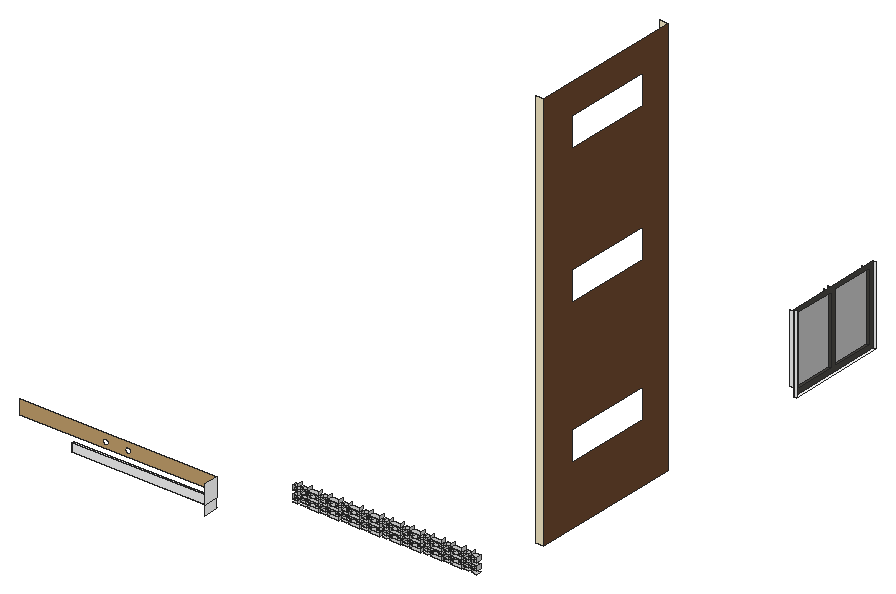
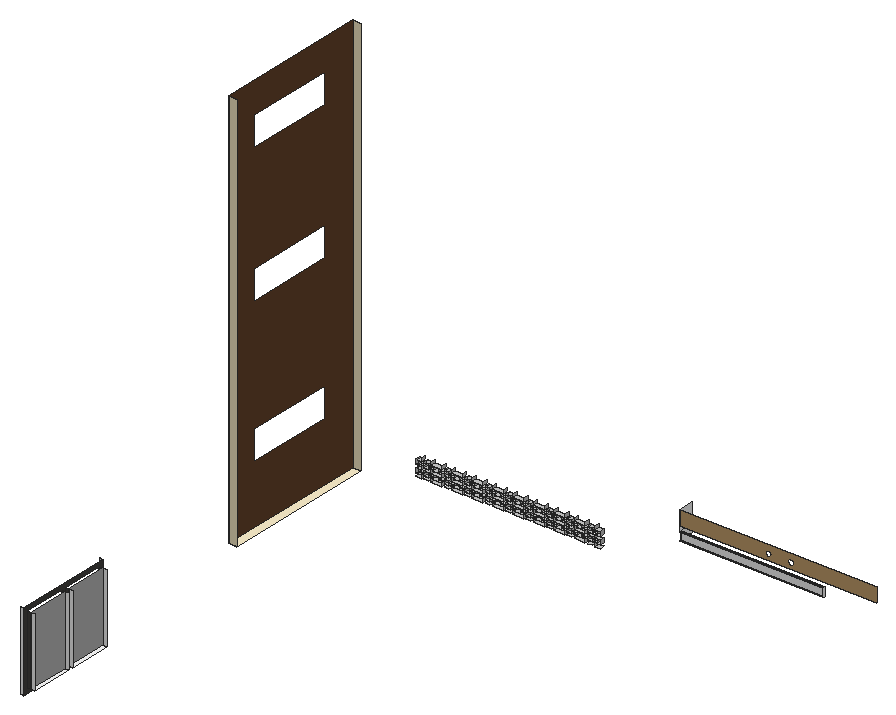
# SketchUp Ruby script. Lengths in inches.
U = 1.inch
M = Sketchup.active_model
def pt(a) = Geom::Point3d.new(a.map { |v| v * U })
def face(e, loops, mat)
  f = e.add_face(loops[0].map { |a| pt(a) })
  loops[1..].each { |l| e.add_face(l.map { |a| pt(a) }).erase! }
  f.material = f.back_material = mat if mat
  f
end
# faces: each face lists its corners as indices into pts; further lists are holes
def faces(e, pts, list, mat = nil) = list.each { |f| face(e, (f[0].is_a?(Array) ? f : [f]).map { |l| l.map { |i| pts[i] } }, mat) }
# xy, xz, yz: faces in a plane at the given z, y or x. An outline is a flat list of corners, or four numbers for a rectangle; further outlines are holes
def ring(l) = l.size == 4 ? [[l[0], l[1]], [l[2], l[1]], [l[2], l[3]], [l[0], l[3]]] : l.each_slice(2).to_a
def flat(e, list, mat, &to3) = list.each { |f| face(e, (f[0].is_a?(Array) ? f : [f]).map { |l| ring(l).map { |u, v| to3.(u, v) } }, mat) }
def xy(e, z, list, mat = nil) = flat(e, list, mat) { |x, y| [x, y, z] }
def xz(e, y, list, mat = nil) = flat(e, list, mat) { |x, z| [x, y, z] }
def yz(e, x, list, mat = nil) = flat(e, list, mat) { |y, z| [x, y, z] }
def lines(e, pts, list) = list.each { |a, b| e.add_line(pt(pts[a]), pt(pts[b])) }
# prism: a flat outline (further loops are holes) pulled along v
def prism(e, loops, v, mat = nil)
  f = face(e, loops, mat); d = Geom::Vector3d.new(v.map { |x| x * U })
  f.pushpull(f.normal.samedirection?(d) ? d.length : -d.length)
end
def box(e, o, s, mat = nil) = prism(e, [[o, [o[0] + s[0], o[1], o[2]], [o[0] + s[0], o[1] + s[1], o[2]], [o[0], o[1] + s[1], o[2]]]], [0, 0, s[2]], mat)
def at(x, y, z, deg = 0) = Geom::Transformation.translation(pt([x, y, z])) * Geom::Transformation.rotation(ORIGIN, Z_AXIS, deg.degrees)
def axes(o, x, y, z) = Geom::Transformation.new([*x, 0, *y, 0, *z, 0, *pt(o).to_a, 1])
def part(name) = M.definitions.add(name)
# library, detail: a bought-in or finely detailed component or shape, given as its bounding box
def library(name, o, s) = part(name).tap { |d| box(d.entities, o, s) }
def detail(e, o, s) = box(e.add_group.entities, o, s)
def put(e, d, t, mat = nil) = e.add_instance(d, t).tap { |i| i.material = mat if mat }
def group(e, t, mat = nil) = e.add_group.tap { |g| g.transformation = t; g.material = mat if mat }.entities
root = M.entities
M.materials.add("D01_Frost_White").color = [255, 242, 206]
M.materials.add("Glass_Mirror_01").color = [185, 185, 185]
M.materials.add("M00_Soft_Cloud").color = [255, 255, 255]
M.materials.add("Metal_Perforated_03_1K").color = [205, 205, 205]
M.materials.add("Plywood_08_1K").color = [202, 166, 113]
M.materials.add("Wood_Planks_01_1K").color = [69, 67, 63]
M.materials.add("Wood_Veneer_15_1K1").color = [103, 69, 45]
xy(root,36.13,[[230.81,76.77,353.54,78.27]],"M00_Soft_Cloud")
xy(root,36.14,[[388.18,115.4375,392.79,119.17],[401.01,115.4375,410.24,119.17],[418.47,115.4375,427.69,119.17],[435.92,115.4375,445.15,119.17],[453.37,115.4375,462.6,119.17],
  [470.82,115.4375,480.05,119.17],[488.27,115.4375,497.5,119.17],[505.72,115.4375,514.95,119.17],[523.18,115.4375,532.4,119.17],[540.63,115.4375,545.24,119.17]],"Metal_Perforated_03_1K")
xy(root,36.25,[[394.84,115.4375,398.97,119.17],[412.29,115.4375,416.42,119.17],[429.74,115.4375,433.87,119.17],[447.19,115.4375,451.32,119.17],[464.65,115.4375,468.77,119.17],
  [482.1,115.4375,486.22,119.17],[499.55,115.4375,503.68,119.17],[517,115.4375,521.13,119.17],[534.45,115.4375,538.58,119.17]],"Metal_Perforated_03_1K")
xy(root,38.1,[[561.28,433.07,564,517.74]],"M00_Soft_Cloud")
xy(root,38.71,[[394.84,115.4375,398.97,119.17],[412.29,115.4375,416.42,119.17],[429.74,115.4375,433.87,119.17],[447.19,115.4375,451.32,119.17],[464.65,115.4375,468.77,119.17],
  [482.1,115.4375,486.22,119.17],[499.55,115.4375,503.68,119.17],[517,115.4375,521.13,119.17],[534.45,115.4375,538.58,119.17]],"Metal_Perforated_03_1K")
xy(root,38.8125,[[388.18,115.4375,392.79,119.17],[401.01,115.4375,410.24,119.17],[418.47,115.4375,427.69,119.17],[435.92,115.4375,445.15,119.17],[453.37,115.4375,462.6,119.17],
  [470.82,115.4375,480.05,119.17],[488.27,115.4375,497.5,119.17],[505.72,115.4375,514.95,119.17],[523.18,115.4375,532.4,119.17],[540.63,115.4375,545.24,119.17]],"Metal_Perforated_03_1K")
xy(root,40.05,[[390.22,115.4375,394.84,119.17],[398.97,115.4375,403.58,119.17],[407.68,115.4375,412.29,119.17],[416.42,115.4375,421.03,119.17],[425.13,115.4375,429.74,119.17],
  [433.87,115.4375,438.48,119.17],[442.58,115.4375,447.19,119.17],[451.32,115.4375,455.93,119.17],[460.03,115.4375,464.65,119.17],[468.77,115.4375,473.39,119.17],
  [477.48,115.4375,482.1,119.17],[486.22,115.4375,490.84,119.17],[494.94,115.4375,499.55,119.17],[503.68,115.4375,508.29,119.17],[512.39,115.4375,517,119.17],
  [521.13,115.4375,525.74,119.17],[529.84,115.4375,534.45,119.17],[538.58,115.4375,543.19,119.17]],"Metal_Perforated_03_1K")
xy(root,41.4,[[390.22,115.4375,394.84,119.17],[398.97,115.4375,403.58,119.17],[407.68,115.4375,412.29,119.17],[416.42,115.4375,421.03,119.17],[425.13,115.4375,429.74,119.17],
  [433.87,115.4375,438.48,119.17],[442.58,115.4375,447.19,119.17],[451.32,115.4375,455.93,119.17],[460.03,115.4375,464.65,119.17],[468.77,115.4375,473.39,119.17],
  [477.48,115.4375,482.1,119.17],[486.22,115.4375,490.84,119.17],[494.94,115.4375,499.55,119.17],[503.68,115.4375,508.29,119.17],[512.39,115.4375,517,119.17],
  [521.13,115.4375,525.74,119.17],[529.84,115.4375,534.45,119.17],[538.58,115.4375,543.19,119.17]],"Metal_Perforated_03_1K")
xy(root,42.1,[[555,437.07,558.14,473.4],[555,477.4,558.14,513.74]],"M00_Soft_Cloud")
xy(root,42.1,[[558.14,437.07,561.28,473.4],[558.14,477.4,561.28,513.74]],"Wood_Planks_01_1K")
xy(root,42.64,[[388.18,115.4375,392.79,119.17],[401.01,115.4375,410.24,119.17],[418.47,115.4375,427.69,119.17],[435.92,115.4375,445.15,119.17],[453.37,115.4375,462.6,119.17],
  [470.82,115.4375,480.05,119.17],[488.27,115.4375,497.5,119.17],[505.72,115.4375,514.95,119.17],[523.18,115.4375,532.4,119.17],[540.63,115.4375,545.24,119.17]],"Metal_Perforated_03_1K")
xy(root,42.74,[[394.84,115.4375,398.97,119.17],[412.29,115.4375,416.42,119.17],[429.74,115.4375,433.87,119.17],[447.19,115.4375,451.32,119.17],[464.65,115.4375,468.77,119.17],
  [482.1,115.4375,486.22,119.17],[499.55,115.4375,503.68,119.17],[517,115.4375,521.13,119.17],[534.45,115.4375,538.58,119.17]],"Metal_Perforated_03_1K")
xy(root,43.27,[[230.81,76.77,353.54,78.27]],"M00_Soft_Cloud")
xy(root,45.2,[[394.84,115.4375,398.97,119.17],[412.29,115.4375,416.42,119.17],[429.74,115.4375,433.87,119.17],[447.19,115.4375,451.32,119.17],[464.65,115.4375,468.77,119.17],
  [482.1,115.4375,486.22,119.17],[499.55,115.4375,503.68,119.17],[517,115.4375,521.13,119.17],[534.45,115.4375,538.58,119.17]],"Metal_Perforated_03_1K")
xy(root,45.31,[[388.18,115.4375,392.79,119.17],[401.01,115.4375,410.24,119.17],[418.47,115.4375,427.69,119.17],[435.92,115.4375,445.15,119.17],[453.37,115.4375,462.6,119.17],
  [470.82,115.4375,480.05,119.17],[488.27,115.4375,497.5,119.17],[505.72,115.4375,514.95,119.17],[523.18,115.4375,532.4,119.17],[540.63,115.4375,545.24,119.17]],"Metal_Perforated_03_1K")
xy(root,46.54,[[390.22,115.4375,394.84,119.17],[398.97,115.4375,403.58,119.17],[407.68,115.4375,412.29,119.17],[416.42,115.4375,421.03,119.17],[425.13,115.4375,429.74,119.17],
  [433.87,115.4375,438.48,119.17],[442.58,115.4375,447.19,119.17],[451.32,115.4375,455.93,119.17],[460.03,115.4375,464.65,119.17],[468.77,115.4375,473.39,119.17],
  [477.48,115.4375,482.1,119.17],[486.22,115.4375,490.84,119.17],[494.94,115.4375,499.55,119.17],[503.68,115.4375,508.29,119.17],[512.39,115.4375,517,119.17],
  [521.13,115.4375,525.74,119.17],[529.84,115.4375,534.45,119.17],[538.58,115.4375,543.19,119.17]],"Metal_Perforated_03_1K")
xy(root,47.9,[[390.22,115.4375,394.84,119.17],[398.97,115.4375,403.58,119.17],[407.68,115.4375,412.29,119.17],[416.42,115.4375,421.03,119.17],[425.13,115.4375,429.74,119.17],
  [433.87,115.4375,438.48,119.17],[442.58,115.4375,447.19,119.17],[451.32,115.4375,455.93,119.17],[460.03,115.4375,464.65,119.17],[468.77,115.4375,473.39,119.17],
  [477.48,115.4375,482.1,119.17],[486.22,115.4375,490.84,119.17],[494.94,115.4375,499.55,119.17],[503.68,115.4375,508.29,119.17],[512.39,115.4375,517,119.17],
  [521.13,115.4375,525.74,119.17],[529.84,115.4375,534.45,119.17],[538.58,115.4375,543.19,119.17]],"Metal_Perforated_03_1K")
xy(root,49.13,[[388.18,115.4375,392.79,119.17],[401.01,115.4375,410.24,119.17],[418.47,115.4375,427.69,119.17],[435.92,115.4375,445.15,119.17],[453.37,115.4375,462.6,119.17],
  [470.82,115.4375,480.05,119.17],[488.27,115.4375,497.5,119.17],[505.72,115.4375,514.95,119.17],[523.18,115.4375,532.4,119.17],[540.63,115.4375,545.24,119.17]],"Metal_Perforated_03_1K")
xy(root,49.23,[[394.84,115.4375,398.97,119.17],[412.29,115.4375,416.42,119.17],[429.74,115.4375,433.87,119.17],[447.19,115.4375,451.32,119.17],[464.65,115.4375,468.77,119.17],
  [482.1,115.4375,486.22,119.17],[499.55,115.4375,503.68,119.17],[517,115.4375,521.13,119.17],[534.45,115.4375,538.58,119.17]],"Metal_Perforated_03_1K")
xy(root,49.46,[[564,154.61,571,286.54]],"D01_Frost_White")
xz(root,76.77,[[230.81,36.13,353.54,43.27]],"M00_Soft_Cloud")
xz(root,78.27,[[[185.54,48,353.54,60],[258.34,50.6,257.72,50.68,257.14,50.92,256.65,51.3,256.27,51.8,256.03,52.38,255.94,53,256.03,53.62,256.27,54.2,256.65,54.7,257.14,55.08,257.72,55.32,258.34,55.4,258.97,55.32,259.54,55.08,260.04,54.7,260.42,54.2,260.66,53.62,260.74,53,260.66,52.38,260.42,51.8,260.04,51.3,259.54,50.92,258.97,50.68],[277.47,50.6,276.85,50.68,276.27,50.92,275.78,51.3,275.39,51.8,275.15,52.38,275.07,53,275.15,53.62,275.39,54.2,275.78,54.7,276.27,55.08,276.85,55.32,277.47,55.4,278.09,55.32,278.67,55.08,279.17,54.7,279.55,54.2,279.79,53.62,279.87,53,279.79,52.38,279.55,51.8,279.17,51.3,278.67,50.92,278.09,50.68]]],"Plywood_08_1K")
xz(root,154.61,[[564,49.46,571,390.99]],"D01_Frost_White")
xz(root,286.54,[[564,49.46,571,390.99]],"D01_Frost_White")
xz(root,433.07,[[561.28,38.1,564,104.83]],"M00_Soft_Cloud")
xz(root,437.07,[[555,42.1,558.14,100.83]],"M00_Soft_Cloud")
xz(root,437.07,[[558.14,42.1,561.28,100.83]],"Wood_Planks_01_1K")
xz(root,473.4,[[555,42.1,558.14,100.83]],"M00_Soft_Cloud")
xz(root,473.4,[[558.14,42.1,561.28,100.83]],"Wood_Planks_01_1K")
xz(root,477.4,[[555,42.1,558.14,100.83]],"M00_Soft_Cloud")
xz(root,477.4,[[558.14,42.1,561.28,100.83]],"Wood_Planks_01_1K")
xz(root,513.74,[[555,42.1,558.14,100.83]],"M00_Soft_Cloud")
xz(root,513.74,[[558.14,42.1,561.28,100.83]],"Wood_Planks_01_1K")
xz(root,517.74,[[561.28,38.1,564,104.83]],"M00_Soft_Cloud")
yz(root,230.81,[[76.77,36.13,78.27,43.27]],"M00_Soft_Cloud")
yz(root,353.54,[[64.77,36.13,76.77,43.27],[64.77,43.27,78.27,60]],"M00_Soft_Cloud")
yz(root,388.18,[[115.4375,38.8125,119.17,42.64],[115.4375,45.31,119.17,49.13]],"Metal_Perforated_03_1K")
yz(root,390.22,[[115.4375,40.05,119.17,41.4],[115.4375,46.54,119.17,47.9]],"Metal_Perforated_03_1K")
yz(root,392.79,[[115.4375,36.14,119.17,38.8125],[115.4375,42.64,119.17,45.31],[115.4375,49.13,119.17,51.8]],"Metal_Perforated_03_1K")
yz(root,394.84,[[115.4375,38.71,119.17,40.05],[115.4375,41.4,119.17,42.74],[115.4375,45.2,119.17,46.54],[115.4375,47.9,119.17,49.23]],"Metal_Perforated_03_1K")
yz(root,398.97,[[115.4375,38.71,119.17,40.05],[115.4375,41.4,119.17,42.74],[115.4375,45.2,119.17,46.54],[115.4375,47.9,119.17,49.23]],"Metal_Perforated_03_1K")
yz(root,401.01,[[115.4375,36.14,119.17,38.8125],[115.4375,42.64,119.17,45.31],[115.4375,49.13,119.17,51.8]],"Metal_Perforated_03_1K")
yz(root,403.58,[[115.4375,40.05,119.17,41.4],[115.4375,46.54,119.17,47.9]],"Metal_Perforated_03_1K")
yz(root,407.68,[[115.4375,40.05,119.17,41.4],[115.4375,46.54,119.17,47.9]],"Metal_Perforated_03_1K")
yz(root,410.24,[[115.4375,36.14,119.17,38.8125],[115.4375,42.64,119.17,45.31],[115.4375,49.13,119.17,51.8]],"Metal_Perforated_03_1K")
yz(root,412.29,[[115.4375,38.71,119.17,40.05],[115.4375,41.4,119.17,42.74],[115.4375,45.2,119.17,46.54],[115.4375,47.9,119.17,49.23]],"Metal_Perforated_03_1K")
yz(root,416.42,[[115.4375,38.71,119.17,40.05],[115.4375,41.4,119.17,42.74],[115.4375,45.2,119.17,46.54],[115.4375,47.9,119.17,49.23]],"Metal_Perforated_03_1K")
yz(root,418.47,[[115.4375,36.14,119.17,38.8125],[115.4375,42.64,119.17,45.31],[115.4375,49.13,119.17,51.8]],"Metal_Perforated_03_1K")
yz(root,421.03,[[115.4375,40.05,119.17,41.4],[115.4375,46.54,119.17,47.9]],"Metal_Perforated_03_1K")
yz(root,425.13,[[115.4375,40.05,119.17,41.4],[115.4375,46.54,119.17,47.9]],"Metal_Perforated_03_1K")
yz(root,427.69,[[115.4375,36.14,119.17,38.8125],[115.4375,42.64,119.17,45.31],[115.4375,49.13,119.17,51.8]],"Metal_Perforated_03_1K")
yz(root,429.74,[[115.4375,38.71,119.17,40.05],[115.4375,41.4,119.17,42.74],[115.4375,45.2,119.17,46.54],[115.4375,47.9,119.17,49.23]],"Metal_Perforated_03_1K")
yz(root,433.87,[[115.4375,38.71,119.17,40.05],[115.4375,41.4,119.17,42.74],[115.4375,45.2,119.17,46.54],[115.4375,47.9,119.17,49.23]],"Metal_Perforated_03_1K")
yz(root,435.92,[[115.4375,36.14,119.17,38.8125],[115.4375,42.64,119.17,45.31],[115.4375,49.13,119.17,51.8]],"Metal_Perforated_03_1K")
yz(root,438.48,[[115.4375,40.05,119.17,41.4],[115.4375,46.54,119.17,47.9]],"Metal_Perforated_03_1K")
yz(root,442.58,[[115.4375,40.05,119.17,41.4],[115.4375,46.54,119.17,47.9]],"Metal_Perforated_03_1K")
yz(root,445.15,[[115.4375,36.14,119.17,38.8125],[115.4375,42.64,119.17,45.31],[115.4375,49.13,119.17,51.8]],"Metal_Perforated_03_1K")
yz(root,447.19,[[115.4375,38.71,119.17,40.05],[115.4375,41.4,119.17,42.74],[115.4375,45.2,119.17,46.54],[115.4375,47.9,119.17,49.23]],"Metal_Perforated_03_1K")
yz(root,451.32,[[115.4375,38.71,119.17,40.05],[115.4375,41.4,119.17,42.74],[115.4375,45.2,119.17,46.54],[115.4375,47.9,119.17,49.23]],"Metal_Perforated_03_1K")
yz(root,453.37,[[115.4375,36.14,119.17,38.8125],[115.4375,42.64,119.17,45.31],[115.4375,49.13,119.17,51.8]],"Metal_Perforated_03_1K")
yz(root,455.93,[[115.4375,40.05,119.17,41.4],[115.4375,46.54,119.17,47.9]],"Metal_Perforated_03_1K")
yz(root,460.03,[[115.4375,40.05,119.17,41.4],[115.4375,46.54,119.17,47.9]],"Metal_Perforated_03_1K")
yz(root,462.6,[[115.4375,36.14,119.17,38.8125],[115.4375,42.64,119.17,45.31],[115.4375,49.13,119.17,51.8]],"Metal_Perforated_03_1K")
yz(root,464.65,[[115.4375,38.71,119.17,40.05],[115.4375,41.4,119.17,42.74],[115.4375,45.2,119.17,46.54],[115.4375,47.9,119.17,49.23]],"Metal_Perforated_03_1K")
yz(root,468.77,[[115.4375,38.71,119.17,40.05],[115.4375,41.4,119.17,42.74],[115.4375,45.2,119.17,46.54],[115.4375,47.9,119.17,49.23]],"Metal_Perforated_03_1K")
yz(root,470.82,[[115.4375,36.14,119.17,38.8125],[115.4375,42.64,119.17,45.31],[115.4375,49.13,119.17,51.8]],"Metal_Perforated_03_1K")
yz(root,473.39,[[115.4375,40.05,119.17,41.4],[115.4375,46.54,119.17,47.9]],"Metal_Perforated_03_1K")
yz(root,477.48,[[115.4375,40.05,119.17,41.4],[115.4375,46.54,119.17,47.9]],"Metal_Perforated_03_1K")
yz(root,480.05,[[115.4375,36.14,119.17,38.8125],[115.4375,42.64,119.17,45.31],[115.4375,49.13,119.17,51.8]],"Metal_Perforated_03_1K")
yz(root,482.1,[[115.4375,38.71,119.17,40.05],[115.4375,41.4,119.17,42.74],[115.4375,45.2,119.17,46.54],[115.4375,47.9,119.17,49.23]],"Metal_Perforated_03_1K")
yz(root,486.22,[[115.4375,38.71,119.17,40.05],[115.4375,41.4,119.17,42.74],[115.4375,45.2,119.17,46.54],[115.4375,47.9,119.17,49.23]],"Metal_Perforated_03_1K")
yz(root,488.27,[[115.4375,36.14,119.17,38.8125],[115.4375,42.64,119.17,45.31],[115.4375,49.13,119.17,51.8]],"Metal_Perforated_03_1K")
yz(root,490.84,[[115.4375,40.05,119.17,41.4],[115.4375,46.54,119.17,47.9]],"Metal_Perforated_03_1K")
yz(root,494.94,[[115.4375,40.05,119.17,41.4],[115.4375,46.54,119.17,47.9]],"Metal_Perforated_03_1K")
yz(root,497.5,[[115.4375,36.14,119.17,38.8125],[115.4375,42.64,119.17,45.31],[115.4375,49.13,119.17,51.8]],"Metal_Perforated_03_1K")
yz(root,499.55,[[115.4375,38.71,119.17,40.05],[115.4375,41.4,119.17,42.74],[115.4375,45.2,119.17,46.54],[115.4375,47.9,119.17,49.23]],"Metal_Perforated_03_1K")
yz(root,503.68,[[115.4375,38.71,119.17,40.05],[115.4375,41.4,119.17,42.74],[115.4375,45.2,119.17,46.54],[115.4375,47.9,119.17,49.23]],"Metal_Perforated_03_1K")
yz(root,505.72,[[115.4375,36.14,119.17,38.8125],[115.4375,42.64,119.17,45.31],[115.4375,49.13,119.17,51.8]],"Metal_Perforated_03_1K")
yz(root,508.29,[[115.4375,40.05,119.17,41.4],[115.4375,46.54,119.17,47.9]],"Metal_Perforated_03_1K")
yz(root,512.39,[[115.4375,40.05,119.17,41.4],[115.4375,46.54,119.17,47.9]],"Metal_Perforated_03_1K")
yz(root,514.95,[[115.4375,36.14,119.17,38.8125],[115.4375,42.64,119.17,45.31],[115.4375,49.13,119.17,51.8]],"Metal_Perforated_03_1K")
yz(root,517,[[115.4375,38.71,119.17,40.05],[115.4375,41.4,119.17,42.74],[115.4375,45.2,119.17,46.54],[115.4375,47.9,119.17,49.23]],"Metal_Perforated_03_1K")
yz(root,521.13,[[115.4375,38.71,119.17,40.05],[115.4375,41.4,119.17,42.74],[115.4375,45.2,119.17,46.54],[115.4375,47.9,119.17,49.23]],"Metal_Perforated_03_1K")
yz(root,523.18,[[115.4375,36.14,119.17,38.8125],[115.4375,42.64,119.17,45.31],[115.4375,49.13,119.17,51.8]],"Metal_Perforated_03_1K")
yz(root,525.74,[[115.4375,40.05,119.17,41.4],[115.4375,46.54,119.17,47.9]],"Metal_Perforated_03_1K")
yz(root,529.84,[[115.4375,40.05,119.17,41.4],[115.4375,46.54,119.17,47.9]],"Metal_Perforated_03_1K")
yz(root,532.4,[[115.4375,36.14,119.17,38.8125],[115.4375,42.64,119.17,45.31],[115.4375,49.13,119.17,51.8]],"Metal_Perforated_03_1K")
yz(root,534.45,[[115.4375,38.71,119.17,40.05],[115.4375,41.4,119.17,42.74],[115.4375,45.2,119.17,46.54],[115.4375,47.9,119.17,49.23]],"Metal_Perforated_03_1K")
yz(root,538.58,[[115.4375,38.71,119.17,40.05],[115.4375,41.4,119.17,42.74],[115.4375,45.2,119.17,46.54],[115.4375,47.9,119.17,49.23]],"Metal_Perforated_03_1K")
yz(root,540.63,[[115.4375,36.14,119.17,38.8125],[115.4375,42.64,119.17,45.31],[115.4375,49.13,119.17,51.8]],"Metal_Perforated_03_1K")
yz(root,543.19,[[115.4375,40.05,119.17,41.4],[115.4375,46.54,119.17,47.9]],"Metal_Perforated_03_1K")
yz(root,545.24,[[115.4375,38.8125,119.17,42.64],[115.4375,45.31,119.17,49.13]],"Metal_Perforated_03_1K")
yz(root,558.14,[[437.07,42.1,473.4,100.83],[477.4,42.1,513.74,100.83]],"Glass_Mirror_01")
yz(root,561.28,[[[433.07,38.1,517.74,104.83],[477.4,42.1,513.74,100.83],[437.07,42.1,473.4,100.83]]],"Wood_Planks_01_1K")
yz(root,571,[[[154.61,49.46,286.54,390.99],[184.64,339.72,259.82,365.04],[184.64,222.33,259.82,247.65],[184.64,99.76,259.82,125.08]]],"Wood_Veneer_15_1K1")
